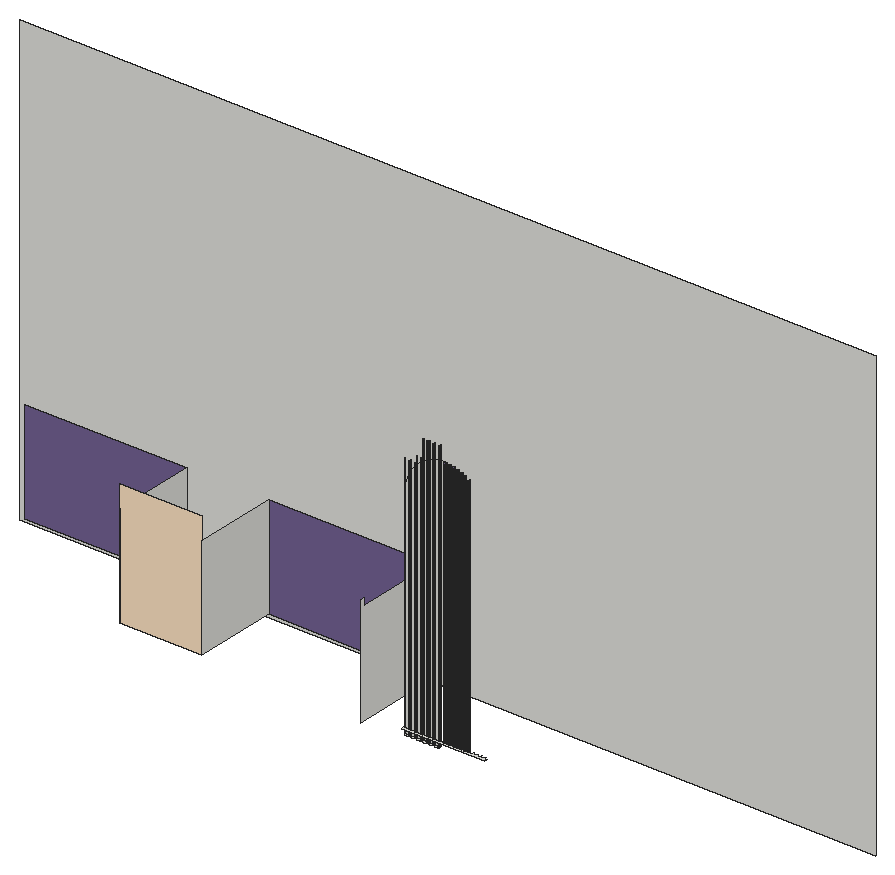
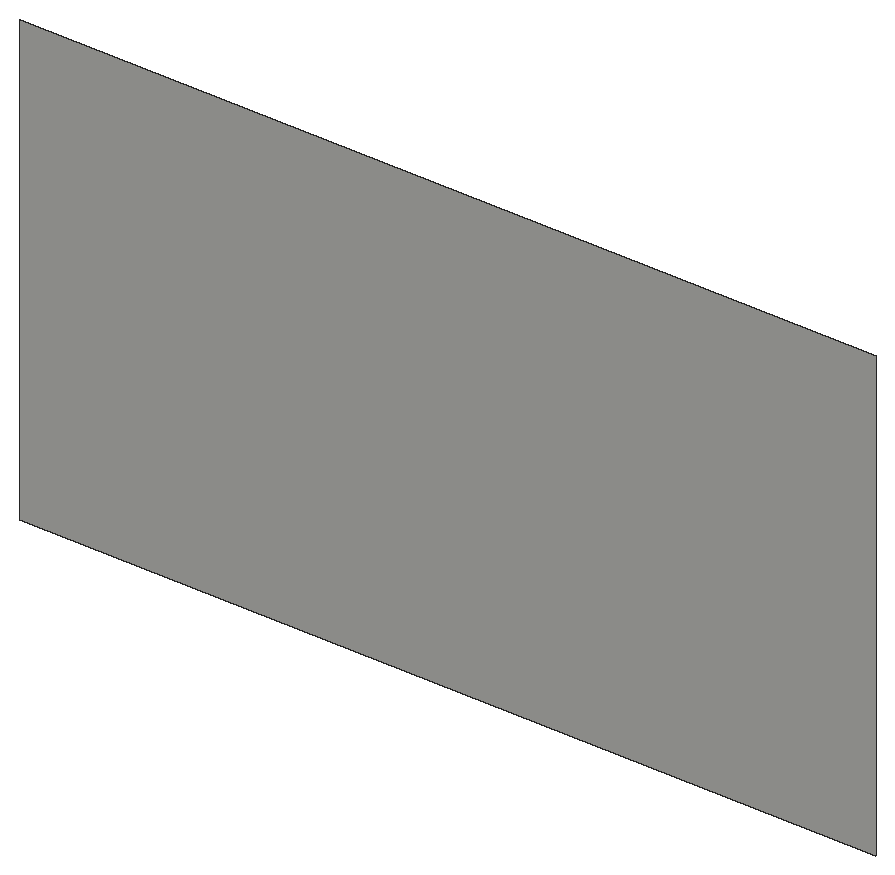
# SketchUp Ruby script. Lengths in inches.
U = 1.inch
M = Sketchup.active_model
def pt(a) = Geom::Point3d.new(a.map { |v| v * U })
def face(e, loops, mat)
  f = e.add_face(loops[0].map { |a| pt(a) })
  loops[1..].each { |l| e.add_face(l.map { |a| pt(a) }).erase! }
  f.material = f.back_material = mat if mat
  f
end
# faces: each face lists its corners as indices into pts; further lists are holes
def faces(e, pts, list, mat = nil) = list.each { |f| face(e, (f[0].is_a?(Array) ? f : [f]).map { |l| l.map { |i| pts[i] } }, mat) }
# xy, xz, yz: faces in a plane at the given z, y or x. An outline is a flat list of corners, or four numbers for a rectangle; further outlines are holes
def ring(l) = l.size == 4 ? [[l[0], l[1]], [l[2], l[1]], [l[2], l[3]], [l[0], l[3]]] : l.each_slice(2).to_a
def flat(e, list, mat, &to3) = list.each { |f| face(e, (f[0].is_a?(Array) ? f : [f]).map { |l| ring(l).map { |u, v| to3.(u, v) } }, mat) }
def xy(e, z, list, mat = nil) = flat(e, list, mat) { |x, y| [x, y, z] }
def xz(e, y, list, mat = nil) = flat(e, list, mat) { |x, z| [x, y, z] }
def yz(e, x, list, mat = nil) = flat(e, list, mat) { |y, z| [x, y, z] }
def lines(e, pts, list) = list.each { |a, b| e.add_line(pt(pts[a]), pt(pts[b])) }
# prism: a flat outline (further loops are holes) pulled along v
def prism(e, loops, v, mat = nil)
  f = face(e, loops, mat); d = Geom::Vector3d.new(v.map { |x| x * U })
  f.pushpull(f.normal.samedirection?(d) ? d.length : -d.length)
end
def box(e, o, s, mat = nil) = prism(e, [[o, [o[0] + s[0], o[1], o[2]], [o[0] + s[0], o[1] + s[1], o[2]], [o[0], o[1] + s[1], o[2]]]], [0, 0, s[2]], mat)
def at(x, y, z, deg = 0) = Geom::Transformation.translation(pt([x, y, z])) * Geom::Transformation.rotation(ORIGIN, Z_AXIS, deg.degrees)
def axes(o, x, y, z) = Geom::Transformation.new([*x, 0, *y, 0, *z, 0, *pt(o).to_a, 1])
def part(name) = M.definitions.add(name)
# library, detail: a bought-in or finely detailed component or shape, given as its bounding box
def library(name, o, s) = part(name).tap { |d| box(d.entities, o, s) }
def detail(e, o, s) = box(e.add_group.entities, o, s)
def put(e, d, t, mat = nil) = e.add_instance(d, t).tap { |i| i.material = mat if mat }
def group(e, t, mat = nil) = e.add_group.tap { |g| g.transformation = t; g.material = mat if mat }.entities
root = M.entities
M.materials.add("[0012_Bisque]").color = [255, 228, 196]
M.materials.add("[Color I01]").color = [116, 98, 147]
xy(root,5.5,[[131.36,140.54,131.29,140.55,131.21,140.57,131.14,140.59,131,140.66,130.93,140.7,130.82,140.8,130.72,140.92,130.68,140.98,130.65,141.05,130.59,141.2,132.28,141.2,132.26,141.125,132.23,141.05,132.2,140.98,132.16,140.92,132.06,140.8,131.94,140.7,131.88,140.66,131.74,140.59,131.67,140.57,131.59,140.55,131.52,140.54],[133.05,140.54,132.97,140.55,132.83,140.59,132.75,140.625,132.6875,140.66,132.62,140.7,132.5625,140.75,132.51,140.8,132.45,140.86,132.37,140.98,132.33,141.05,132.3,141.125,132.28,141.2,133.97,141.2,133.95,141.125,133.92,141.05,133.88,140.98,133.8,140.86,133.75,140.8,133.63,140.7,133.57,140.66,133.43,140.59,133.35,140.57,133.28,140.55,133.2,140.54],[134.74,140.54,134.66,140.55,134.59,140.57,134.51,140.59,134.44,140.625,134.375,140.66,134.31,140.7,134.19,140.8,134.14,140.86,134.06,140.98,134.02,141.05,133.99,141.125,133.97,141.2,135.66,141.2,135.64,141.125,135.61,141.05,135.57,140.98,135.49,140.86,135.38,140.75,135.32,140.7,135.25,140.66,135.11,140.59,134.97,140.55,134.89,140.54],[136.42,140.54,136.35,140.55,136.27,140.57,136.2,140.59,136.13,140.625,136.0625,140.66,136,140.7,135.9375,140.75,135.88,140.8,135.78,140.92,135.74,140.98,135.71,141.05,135.68,141.125,135.66,141.2,137.28,141.2,137.3,141.125,137.3125,141.1,137.29,141.05,137.26,140.98,137.22,140.92,137.12,140.8,137.07,140.75,137,140.7,136.94,140.66,136.8,140.59,136.73,140.57,136.65,140.55,136.58,140.54],[138.05,140.54,137.97,140.55,137.83,140.59,137.75,140.625,137.6875,140.66,137.62,140.7,137.5625,140.75,137.51,140.8,137.45,140.86,137.37,140.98,137.33,141.05,137.3125,141.1,137.32,141.125,137.34,141.2,138.91,141.2,138.93,141.125,138.9375,141.1,138.92,141.05,138.88,140.98,138.8,140.86,138.75,140.8,138.63,140.7,138.57,140.66,138.43,140.59,138.35,140.57,138.28,140.55,138.2,140.54],
  [139.67,140.54,139.6,140.55,139.52,140.57,139.45,140.59,139.38,140.625,139.3125,140.66,139.25,140.7,139.1875,140.75,139.13,140.8,139.03,140.92,138.99,140.98,138.96,141.05,138.9375,141.1,138.95,141.125,138.97,141.2,140.53,141.2,140.55,141.125,140.5625,141.1,140.54,141.05,140.51,140.98,140.47,140.92,140.37,140.8,140.32,140.75,140.25,140.7,140.19,140.66,140.05,140.59,139.98,140.57,139.9,140.55,139.83,140.54],[137.3125,141.1,137.32,141.125,137.34,141.2,137.28,141.2,137.3,141.125],[138.9375,141.1,138.95,141.125,138.97,141.2,138.91,141.2,138.93,141.125],[140.5625,141.1,140.57,141.125,140.59,141.2,140.53,141.2,140.55,141.125]])
xy(root,7.1875,[[130.59,139.88,153.72,139.88,153.72,140.74,153.6,140.68,153.46,140.67,153.32,140.68,153.19,140.74,153.08,140.82,153,140.93,152.95,141.06,152.93,141.2,152.91,141.06,152.86,140.93,152.77,140.82,152.66,140.74,152.53,140.68,152.4,140.67,152.26,140.68,152.13,140.74,152.02,140.82,151.9375,140.93,151.88,141.06,151.86,141.2,151.85,141.06,151.79,140.93,151.71,140.82,151.6,140.74,151.47,140.68,151.33,140.67,151.2,140.68,151.07,140.74,150.96,140.82,150.875,140.93,150.82,141.06,150.8,141.2,150.78,141.06,150.73,140.93,150.65,140.82,150.54,140.74,150.41,140.68,150.27,140.67,150.13,140.68,150.01,140.74,149.9,140.82,149.8125,140.93,149.76,141.06,149.74,141.2,149.72,141.06,149.67,140.93,149.58,140.82,149.47,140.74,149.35,140.68,149.21,140.67,149.07,140.68,148.94,140.74,148.83,140.82,148.75,140.93,148.7,141.06,148.68,141.2,148.66,141.06,148.61,140.93,148.52,140.82,148.41,140.74,148.28,140.68,148.15,140.67,148.01,140.68,147.88,140.74,147.77,140.82,147.6875,140.93,147.63,141.06,147.61,141.2,147.6,141.06,147.54,140.93,147.46,140.82,147.35,140.74,147.22,140.68,147.08,140.67,146.95,140.68,146.82,140.74,146.71,140.82,146.625,140.93,146.57,141.06,146.55,141.2,146.53,141.06,146.48,140.93,146.4,140.82,146.29,140.74,146.16,140.68,146.02,140.67,145.88,140.68,145.76,140.74,145.65,140.82,145.5625,140.93,145.51,141.06,145.49,141.2,145.47,141.06,145.42,140.93,145.33,140.82,145.22,140.74,145.1,140.68,144.96,140.67,144.82,140.68,144.69,140.74,144.58,140.82,144.5,140.93,144.45,141.06,144.43,141.2,144.41,141.06,144.36,140.93,144.27,140.82,144.16,140.74,144.03,140.68,143.9,140.67,143.76,140.68,143.63,140.74,143.52,140.82,143.4375,140.93,143.38,141.06,143.36,141.2,143.35,141.06,143.29,140.93,143.21,140.82,143.1,140.74,142.97,140.68,142.83,140.67,142.7,140.68,142.57,140.74,142.46,140.82,142.375,140.93,142.32,141.06,142.3,141.2,142,141.2,141.96,141.04,141.875,140.9,141.77,140.78,141.63,140.68,141.48,140.62,141.32,140.59,141.16,140.6,141,140.64,140.85,140.71,140.73,140.82,140.63,140.95,140.5625,141.1,140.54,141.05,140.51,140.98,140.47,140.92,140.37,140.8,140.32,140.75,140.25,140.7,140.19,140.66,140.05,140.59,139.98,140.57,139.9,140.55,139.83,140.54,139.67,140.54,139.6,140.55,139.52,140.57,139.45,140.59,139.38,140.625,139.3125,140.66,139.25,140.7,139.1875,140.75,139.13,140.8,139.03,140.92,138.99,140.98,138.96,141.05,138.9375,141.1,138.92,141.05,138.88,140.98,138.8,140.86,138.75,140.8,138.63,140.7,138.57,140.66,138.43,140.59,138.35,140.57,138.28,140.55,138.2,140.54,138.05,140.54,137.97,140.55,137.83,140.59,137.75,140.625,137.6875,140.66,137.62,140.7,137.5625,140.75,137.51,140.8,137.45,140.86,137.37,140.98,137.33,141.05,137.3125,141.1,137.29,141.05,137.26,140.98,137.22,140.92,137.12,140.8,137.07,140.75,137,140.7,136.94,140.66,136.8,140.59,136.73,140.57,136.65,140.55,136.58,140.54,136.42,140.54,136.35,140.55,136.27,140.57,136.2,140.59,136.13,140.625,136.0625,140.66,136,140.7,135.9375,140.75,135.88,140.8,135.78,140.92,135.74,140.98,135.71,141.05,135.68,141.125,135.66,141.2,135.64,141.125,135.61,141.05,135.57,140.98,135.49,140.86,135.38,140.75,135.32,140.7,135.25,140.66,135.11,140.59,134.97,140.55,134.89,140.54,134.74,140.54,134.66,140.55,134.59,140.57,134.51,140.59,134.44,140.625,134.375,140.66,134.31,140.7,134.19,140.8,134.14,140.86,134.06,140.98,134.02,141.05,133.99,141.125,133.97,141.2,133.95,141.125,133.92,141.05,133.88,140.98,133.8,140.86,133.75,140.8,133.63,140.7,133.57,140.66,133.43,140.59,133.35,140.57,133.28,140.55,133.2,140.54,133.05,140.54,132.97,140.55,132.83,140.59,132.75,140.625,132.6875,140.66,132.62,140.7,132.5625,140.75,132.51,140.8,132.45,140.86,132.37,140.98,132.33,141.05,132.3,141.125,132.28,141.2,132.26,141.125,132.23,141.05,132.2,140.98,132.16,140.92,132.06,140.8,131.94,140.7,131.88,140.66,131.74,140.59,131.67,140.57,131.59,140.55,131.52,140.54,131.36,140.54,131.29,140.55,131.21,140.57,131.14,140.59,131,140.66,130.93,140.7,130.82,140.8,130.72,140.92,130.68,140.98,130.65,141.05,130.59,141.2]])
xz(root,141.2,[[130.59,5.5,132.28,5.5,132.28,71.42,132.27,71.4,132.12,71.15,131.97,70.88,131.83,70.62,131.7,70.35,131.58,70.07,131.46,69.8,131.35,69.52,131.25,69.24,131.15,68.95,131.0625,68.67,130.98,68.38,130.91,68.09,130.84,67.79,130.79,67.5,130.73,67.2,130.69,66.91,130.63,66.31,130.61,66.01,130.59,65.41],[132.28,5.5,133.97,5.5,133.97,73.57,133.93,73.53,133.72,73.3125,133.52,73.09,133.32,72.87,133.13,72.63,132.94,72.4,132.77,72.16,132.59,71.91,132.43,71.66,132.28,71.42],[133.97,5.5,135.66,5.5,135.66,74.97,135.53,74.88,135.29,74.71,135.05,74.53,134.8125,74.34,134.58,74.15,134.36,73.95,134.14,73.74,133.97,73.57],[135.66,5.5,137.28,5.5,137.28,75.89,137.08,75.8,136.8125,75.66,136.55,75.52,136.03,75.22,135.78,75.05,135.66,74.97],[137.28,5.5,137.34,5.5,137.34,75.92,137.28,75.89],
  [137.34,5.5,138.91,5.5,138.91,76.5,138.75,76.46,138.47,76.37,138.18,76.27,137.9,76.16,137.625,76.05,137.35,75.93,137.34,75.92],[138.91,5.5,138.97,5.5,138.97,76.52,138.91,76.5],[138.97,5.5,140.53,5.5,140.53,76.86,140.51,76.85,140.21,76.81,139.92,76.75,139.62,76.69,139.33,76.62,139.04,76.54,138.97,76.52],[140.53,5.5,140.59,5.5,140.59,76.87,142,76.87,142,76.95,141.7,76.96,141.4,76.95,140.8,76.89,140.59,76.87,140.53,76.86],[142,7.1875,142.3,7.1875,142.3,76.97,142,76.95]])
xz(root,141.7,[[50.74,4.6875,73.56,39.45]],"[0012_Bisque]")
xz(root,164.88,[[5.62,4.6875,50.74,33.18],[73.56,4.6875,119.1875,33.18]],"[Color I01]")
xz(root,170.3125,[[0,0,238.375,124.6875]])
yz(root,50.74,[[141.7,4.6875,164.88,33.18]])
yz(root,73.56,[[141.7,4.6875,164.88,33.18]])
yz(root,119.1875,[[139.88,4.6875,139.88,35.18,141.2,35.18,141.2,33.18,164.88,33.18,164.88,4.6875]])
p = [[133.69,140.75,5.5],[133.75,140.8,5.5],[133.75,140.8,7.1875],[133.69,140.75,7.1875],[134.19,140.8,5.5],[134.25,140.75,5.5],
  [134.25,140.75,7.1875],[134.19,140.8,7.1875],[135.38,140.75,5.5],[135.43,140.8,5.5],[135.43,140.8,7.1875],[135.38,140.75,7.1875],
  [135.88,140.8,5.5],[135.9375,140.75,5.5],[135.9375,140.75,7.1875],[135.88,140.8,7.1875],[137.07,140.75,5.5],[137.12,140.8,5.5],
  [137.12,140.8,7.1875],[137.07,140.75,7.1875],[137.51,140.8,5.5],[137.5625,140.75,5.5],[137.5625,140.75,7.1875],[137.51,140.8,7.1875],
  [138.69,140.75,5.5],[138.75,140.8,5.5],[138.75,140.8,7.1875],[138.69,140.75,7.1875],[139.13,140.8,5.5],[139.1875,140.75,5.5],
  [139.1875,140.75,7.1875],[139.13,140.8,7.1875],[140.32,140.75,5.5],[140.37,140.8,5.5],[140.37,140.8,7.1875],[140.32,140.75,7.1875],
  [130.77,140.86,5.5],[130.82,140.8,5.5],[130.82,140.8,7.1875],[130.77,140.86,7.1875],[132.06,140.8,5.5],[132.11,140.86,5.5],
  [132.11,140.86,7.1875],[132.06,140.8,7.1875],[132.45,140.86,5.5],[132.51,140.8,5.5],[132.51,140.8,7.1875],[132.45,140.86,7.1875],
  [133.8,140.86,5.5],[133.8,140.86,7.1875],[134.14,140.86,5.5],[134.14,140.86,7.1875],[135.49,140.86,5.5],[135.49,140.86,7.1875],
  [135.83,140.86,5.5],[135.83,140.86,7.1875],[137.17,140.86,5.5],[137.17,140.86,7.1875],[137.45,140.86,5.5],[137.45,140.86,7.1875],
  [138.8,140.86,5.5],[138.8,140.86,7.1875],[139.08,140.86,5.5],[139.08,140.86,7.1875],[140.42,140.86,5.5],[140.42,140.86,7.1875],
  [130.72,140.92,5.5],[130.72,140.92,7.1875],[130.68,140.98,5.5],[130.68,140.98,7.1875],[132.16,140.92,5.5],[132.16,140.92,7.1875],
  [132.2,140.98,5.5],[132.2,140.98,7.1875],[132.41,140.92,5.5],[132.41,140.92,7.1875],[132.37,140.98,5.5],[132.37,140.98,7.1875],
  [133.84,140.92,5.5],[133.84,140.92,7.1875],[133.88,140.98,5.5],[133.88,140.98,7.1875],[134.1,140.92,5.5],[134.1,140.92,7.1875],
  [134.06,140.98,5.5],[134.06,140.98,7.1875],[135.53,140.92,5.5],[135.53,140.92,7.1875],[135.57,140.98,5.5],[135.57,140.98,7.1875],
  [135.74,140.98,5.5],[135.78,140.92,5.5],[135.78,140.92,7.1875],[135.74,140.98,7.1875],[137.22,140.92,5.5],[137.22,140.92,7.1875],
  [137.26,140.98,5.5],[137.26,140.98,7.1875],[137.41,140.92,5.5],[137.41,140.92,7.1875],[137.37,140.98,5.5],[137.37,140.98,7.1875],
  [138.84,140.92,5.5],[138.84,140.92,7.1875],[138.88,140.98,5.5],[138.88,140.98,7.1875],[139.03,140.92,5.5],[139.03,140.92,7.1875],
  [138.99,140.98,5.5],[138.99,140.98,7.1875],[140.47,140.92,5.5],[140.47,140.92,7.1875],[140.51,140.98,5.5],[140.51,140.98,7.1875],
  [130.65,141.05,5.5],[130.65,141.05,7.1875],[132.23,141.05,5.5],[132.23,141.05,7.1875],[132.33,141.05,5.5],[132.33,141.05,7.1875],
  [133.92,141.05,5.5],[133.92,141.05,7.1875],[134.02,141.05,5.5],[134.02,141.05,7.1875],[135.61,141.05,5.5],[135.61,141.05,7.1875],
  [135.71,141.05,5.5],[135.71,141.05,7.1875],[137.29,141.05,5.5],[137.29,141.05,7.1875],[137.33,141.05,5.5],[137.33,141.05,7.1875],
  [138.92,141.05,5.5],[138.92,141.05,7.1875],[138.96,141.05,5.5],[138.96,141.05,7.1875],[140.54,141.05,5.5],[140.54,141.05,7.1875],
  [130.62,141.125,5.5],[130.62,141.125,7.1875],[130.59,141.2,5.5],[130.59,141.2,7.1875],[132.26,141.125,5.5],[132.26,141.125,7.1875],
  [132.3,141.125,5.5],[132.3,141.125,7.1875],[132.28,141.2,5.5],[132.28,141.2,7.1875],[133.95,141.125,5.5],[133.95,141.125,7.1875],
  [133.97,141.2,5.5],[133.97,141.2,7.1875],[133.99,141.125,5.5],[133.99,141.125,7.1875],[135.64,141.125,5.5],[135.64,141.125,7.1875],
  [135.66,141.2,5.5],[135.66,141.2,7.1875],[135.68,141.125,5.5],[135.68,141.125,7.1875],[137.3125,141.1,5.5],[137.3125,141.1,7.1875],
  [137.3,141.125,5.5],[137.3,141.125,80.75],[137.3125,141.1,80.75],[137.32,141.125,5.5],[137.32,141.125,80.75],[137.28,141.2,5.5],
  [137.28,141.2,75.89],[137.28,141.2,80.75],[137.34,141.2,5.5],[137.34,141.2,80.75],[137.34,141.2,75.92],[138.9375,141.1,5.5],
  [138.9375,141.1,7.1875],[138.93,141.125,5.5],[138.93,141.125,80.75],[138.9375,141.1,80.75],[138.95,141.125,5.5],[138.95,141.125,80.75],
  [138.91,141.2,5.5],[138.91,141.2,76.5],[138.91,141.2,80.75],[138.97,141.2,5.5],[138.97,141.2,80.75],[138.97,141.2,76.52],
  [140.5625,141.1,5.5],[140.5625,141.1,7.1875],[140.55,141.125,5.5],[140.53,141.2,5.5],[140.53,141.2,76.86],[140.53,141.2,80.75],
  [140.55,141.125,80.75],[140.5625,141.1,80.75],[140.5625,141.1,76.87],[140.57,141.125,5.5],[140.57,141.125,76.87],[140.59,141.2,5.5],
  [140.59,141.2,76.87],[132.51,140.8,74.15],[132.5625,140.75,7.1875],[132.5625,140.75,74.15],[133.69,140.75,74.15],[133.75,140.8,74.15],
  [134.19,140.8,75.9375],[134.25,140.75,75.9375],[135.38,140.75,75.9375],[135.43,140.8,75.9375],[135.88,140.8,80.75],[135.9375,140.75,80.75],
  [137.07,140.75,80.75],[137.12,140.8,80.75],[137.51,140.8,80.75],[137.5625,140.75,80.75],[138.69,140.75,80.75],[138.75,140.8,80.75],
  [139.13,140.8,80.75],[139.1875,140.75,80.75],[140.32,140.75,80.75],[140.37,140.8,80.75],[142.46,140.82,76.91],[142.46,140.82,7.1875],
  [142.57,140.74,7.1875],[142.57,140.74,76.91],[143.1,140.74,76.91],[143.1,140.74,7.1875],[143.21,140.82,7.1875],[143.21,140.82,76.91],
  [143.52,140.82,76.75],[143.52,140.82,7.1875],[143.63,140.74,7.1875],[143.63,140.74,76.75],[144.16,140.74,76.75],[144.16,140.74,7.1875],
  [144.27,140.82,7.1875],[144.27,140.82,76.75],[144.58,140.82,76.48],[144.58,140.82,7.1875],[144.69,140.74,7.1875],[144.69,140.74,76.48],
  [145.22,140.74,76.48],[145.22,140.74,7.1875],[145.33,140.82,7.1875],[145.33,140.82,76.48],[145.65,140.82,76.1],[145.65,140.82,7.1875],
  [145.76,140.74,7.1875],[145.76,140.74,76.1],[146.29,140.74,76.1],[146.29,140.74,7.1875],[146.4,140.82,7.1875],[146.4,140.82,76.1],
  [146.71,140.82,75.6],[146.71,140.82,7.1875],[146.82,140.74,7.1875],[146.82,140.74,75.6],[147.35,140.74,75.6],[147.35,140.74,7.1875],
  [147.46,140.82,7.1875],[147.46,140.82,75.6],[147.77,140.82,74.96],[147.77,140.82,7.1875],[147.88,140.74,7.1875],[147.88,140.74,74.96],
  [148.41,140.74,74.96],[148.41,140.74,7.1875],[148.52,140.82,7.1875],[148.52,140.82,74.96],[130.77,140.86,74.15],[130.82,140.8,74.15],
  [132.06,140.8,74.15],[132.11,140.86,74.15],[132.45,140.86,74.15],[133.8,140.86,74.15],[134.14,140.86,75.9375],[135.49,140.86,75.9375],
  [135.83,140.86,80.75],[137.17,140.86,80.75],[137.45,140.86,80.75],[138.8,140.86,80.75],[139.08,140.86,80.75],[140.42,140.86,80.75],
  [140.63,140.95,76.87],[140.63,140.95,7.1875],[140.73,140.82,7.1875],[140.73,140.82,76.87],[141.77,140.78,76.87],[141.77,140.78,7.1875],
  [141.875,140.9,7.1875],[141.875,140.9,76.87],[142.375,140.93,76.91],[142.375,140.93,7.1875],[143.29,140.93,7.1875],[143.29,140.93,76.91],
  [143.4375,140.93,76.75],[143.4375,140.93,7.1875],[144.36,140.93,7.1875],[144.36,140.93,76.75],[144.5,140.93,76.48],[144.5,140.93,7.1875],
  [145.42,140.93,7.1875],[145.42,140.93,76.48],[145.5625,140.93,76.1],[145.5625,140.93,7.1875],[146.48,140.93,7.1875],[146.48,140.93,76.1],
  [146.625,140.93,75.6],[146.625,140.93,7.1875],[147.54,140.93,7.1875],[147.54,140.93,75.6],[147.6875,140.93,74.96],[147.6875,140.93,7.1875],
  [148.61,140.93,7.1875],[148.61,140.93,74.96],[130.72,140.92,74.15],[130.68,140.98,74.15],[132.16,140.92,74.15],[132.2,140.98,74.15],
  [132.41,140.92,74.15],[132.37,140.98,74.15],[133.84,140.92,74.15],[133.88,140.98,74.15],[134.1,140.92,75.9375],[134.06,140.98,75.9375],
  [135.53,140.92,75.9375],[135.57,140.98,75.9375],[135.74,140.98,80.75],[135.78,140.92,80.75],[137.22,140.92,80.75],[137.26,140.98,80.75],
  [137.41,140.92,80.75],[137.37,140.98,80.75],[138.84,140.92,80.75],[138.88,140.98,80.75],[139.03,140.92,80.75],[138.99,140.98,80.75],
  [140.47,140.92,80.75],[140.51,140.98,80.75],[141.96,141.04,7.1875],[141.96,141.04,76.87],[142.32,141.06,76.91],[142.32,141.06,7.1875],
  [143.35,141.06,7.1875],[143.35,141.06,76.91],[143.38,141.06,76.75],[143.38,141.06,7.1875],[144.41,141.06,7.1875],[144.41,141.06,76.75],
  [144.45,141.06,76.48],[144.45,141.06,7.1875],[145.47,141.06,7.1875],[145.47,141.06,76.48],[145.51,141.06,76.1],[145.51,141.06,7.1875],
  [146.53,141.06,7.1875],[146.53,141.06,76.1],[146.57,141.06,75.6],[146.57,141.06,7.1875],[147.6,141.06,7.1875],[147.6,141.06,75.6],
  [147.63,141.06,74.96],[147.63,141.06,7.1875],[148.66,141.06,7.1875],[148.66,141.06,74.96],[130.65,141.05,74.15],[132.23,141.05,74.15],
  [132.33,141.05,74.15],[133.92,141.05,74.15],[134.02,141.05,75.9375],[135.61,141.05,75.9375],[135.71,141.05,80.75],[137.29,141.05,80.75],
  [137.33,141.05,80.75],[138.92,141.05,80.75],[138.96,141.05,80.75],[140.54,141.05,80.75],[142,141.2,7.1875],[142,141.2,76.87],
  [130.62,141.125,74.15],[130.59,141.2,65.41],[130.59,141.2,74.15],[132.26,141.125,74.15],[132.3,141.125,74.15],[132.28,141.2,71.42],
  [132.28,141.2,74.15],[133.95,141.125,74.15],[133.97,141.2,73.57],[133.97,141.2,74.15],[133.99,141.125,75.9375],[133.97,141.2,75.9375],
  [135.64,141.125,75.9375],[135.66,141.2,74.97],[135.66,141.2,75.9375],[135.68,141.125,80.75],[135.66,141.2,80.75],[142.3,141.2,76.91],
  [142.3,141.2,7.1875],[143.36,141.2,7.1875],[143.36,141.2,76.75],[143.36,141.2,76.91],[144.43,141.2,76.48],[144.43,141.2,7.1875],
  [144.43,141.2,76.75],[145.49,141.2,76.1],[145.49,141.2,7.1875],[145.49,141.2,76.48],[146.55,141.2,7.1875],[146.55,141.2,75.6],
  [146.55,141.2,76.1],[147.61,141.2,74.96],[147.61,141.2,7.1875],[147.61,141.2,75.6],[148.68,141.2,7.1875],[148.68,141.2,74.14],
  [148.68,141.2,74.96]]
faces(root,p,[[0,1,2,3],[4,5,6,7],[8,9,10,11],[12,13,14,15],[16,17,18,19],[20,21,22,23],[24,25,26,27],[28,29,30,31],
  [32,33,34,35],[36,37,38,39],[40,41,42,43],[44,45,46,47],[1,48,49,2],[50,4,7,51],[9,52,53,10],[54,12,15,55],
  [17,56,57,18],[58,20,23,59],[25,60,61,26],[62,28,31,63],[33,64,65,34],[66,36,39,67],[68,66,67,69],[41,70,71,42],
  [70,72,73,71],[74,44,47,75],[76,74,75,77],[48,78,79,49],[78,80,81,79],[82,50,51,83],[84,82,83,85],[52,86,87,53],
  [86,88,89,87],[90,91,92,93],[91,54,55,92],[56,94,95,57],[94,96,97,95],[98,58,59,99],[100,98,99,101],[60,102,103,61],
  [102,104,105,103],[106,62,63,107],[108,106,107,109],[64,110,111,65],[110,112,113,111],[114,68,69,115],[72,116,117,73],[118,76,77,119],
  [80,120,121,81],[122,84,85,123],[88,124,125,89],[126,90,93,127],[96,128,129,97],[130,100,101,131],[104,132,133,105],[134,108,109,135],
  [112,136,137,113],[138,114,115,139],[140,138,139,141],[116,142,143,117],[144,118,119,145],[142,146,147,143],[146,144,145,147],[120,148,149,121],
  [148,150,151,149],[152,122,123,153],[150,152,153,151],[124,154,155,125],[154,156,157,155],[158,126,127,159],[156,158,159,157],[128,160,161,129],
  [160,130,131,161],[160,162,163,164,161],[165,160,161,164,166],[162,167,168,169,163],[170,165,166,171,172],[132,173,174,133],[173,134,135,174],[173,175,176,177,174],
  [178,173,174,177,179],[175,180,181,182,176],[183,178,179,184,185],[136,186,187,137],[188,189,190,191,192],[186,188,192,193,194,187],[195,186,187,194,196],[197,195,196,198]])
faces(root,p,[[199,46,200,201],[202,3,2,203],[204,7,6,205],[206,11,10,207],[208,15,14,209],[210,19,18,211],[212,23,22,213],[214,27,26,215],
  [216,31,30,217],[218,35,34,219],[220,221,222,223],[224,225,226,227],[228,229,230,231],[232,233,234,235],[236,237,238,239],[240,241,242,243],
  [244,245,246,247],[248,249,250,251],[252,253,254,255],[256,257,258,259],[260,261,262,263],[264,265,266,267],[268,39,38,269],[270,43,42,271],
  [272,47,46,199],[203,2,49,273],[274,51,7,204],[207,10,53,275],[276,55,15,208],[211,18,57,277],[278,59,23,212],[215,26,61,279],
  [280,63,31,216],[219,34,65,281],[282,283,284,285],[286,287,288,289],[290,291,221,220],[227,226,292,293],[294,295,229,228],[235,234,296,297],
  [298,299,237,236],[243,242,300,301],[302,303,245,244],[251,250,304,305],[306,307,253,252],[259,258,308,309],[310,311,261,260],[267,266,312,313],
  [314,67,39,268],[315,69,67,314],[271,42,71,316],[316,71,73,317],[318,75,47,272],[319,77,75,318],[273,49,79,320],[320,79,81,321],
  [322,83,51,274],[323,85,83,322],[275,53,87,324],[324,87,89,325],[326,93,92,327],[327,92,55,276],[277,57,95,328],[328,95,97,329],
  [330,99,59,278],[331,101,99,330],[279,61,103,332],[332,103,105,333],[334,107,63,280],[335,109,107,334],[281,65,111,336],[336,111,113,337],
  [289,288,338,339],[340,341,291,290],[293,292,342,343],[344,345,295,294],[297,296,346,347],[348,349,299,298],[301,300,350,351],[352,353,303,302],
  [305,304,354,355],[356,357,307,306],[309,308,358,359],[360,361,311,310],[313,312,362,363],[364,115,69,315],[317,73,117,365],[366,119,77,319],
  [321,81,121,367],[368,123,85,323],[325,89,125,369],[370,127,93,326],[329,97,129,371],[372,131,101,331],[333,105,133,373],[374,135,109,335],
  [337,113,137,375],[194,187,283,282],[339,338,376,377],[378,139,115,364],[379,141,139,378,380],[365,117,143,381],[382,145,119,366],[381,143,147,383,384],
  [383,147,145,382,384],[367,121,149,385],[385,149,151,386,387],[388,153,123,368],[386,151,153,388,389,387],[369,125,155,390],[390,155,157,391,392],[393,159,127,370],
  [391,157,159,393,394,392],[371,129,161,164],[164,161,131,372],[373,133,174,177],[177,174,135,374],[375,137,187,194,193],[395,396,341,340],[343,342,397,398,399],
  [398,397,345,344],[400,401,349,348],[347,346,401,400,402],[403,404,353,352],[351,350,404,403,405],[355,354,406,407,408],[407,406,357,356],[409,410,361,360],
  [359,358,410,409,411],[363,362,412,413,414]],"[Color I01]")
